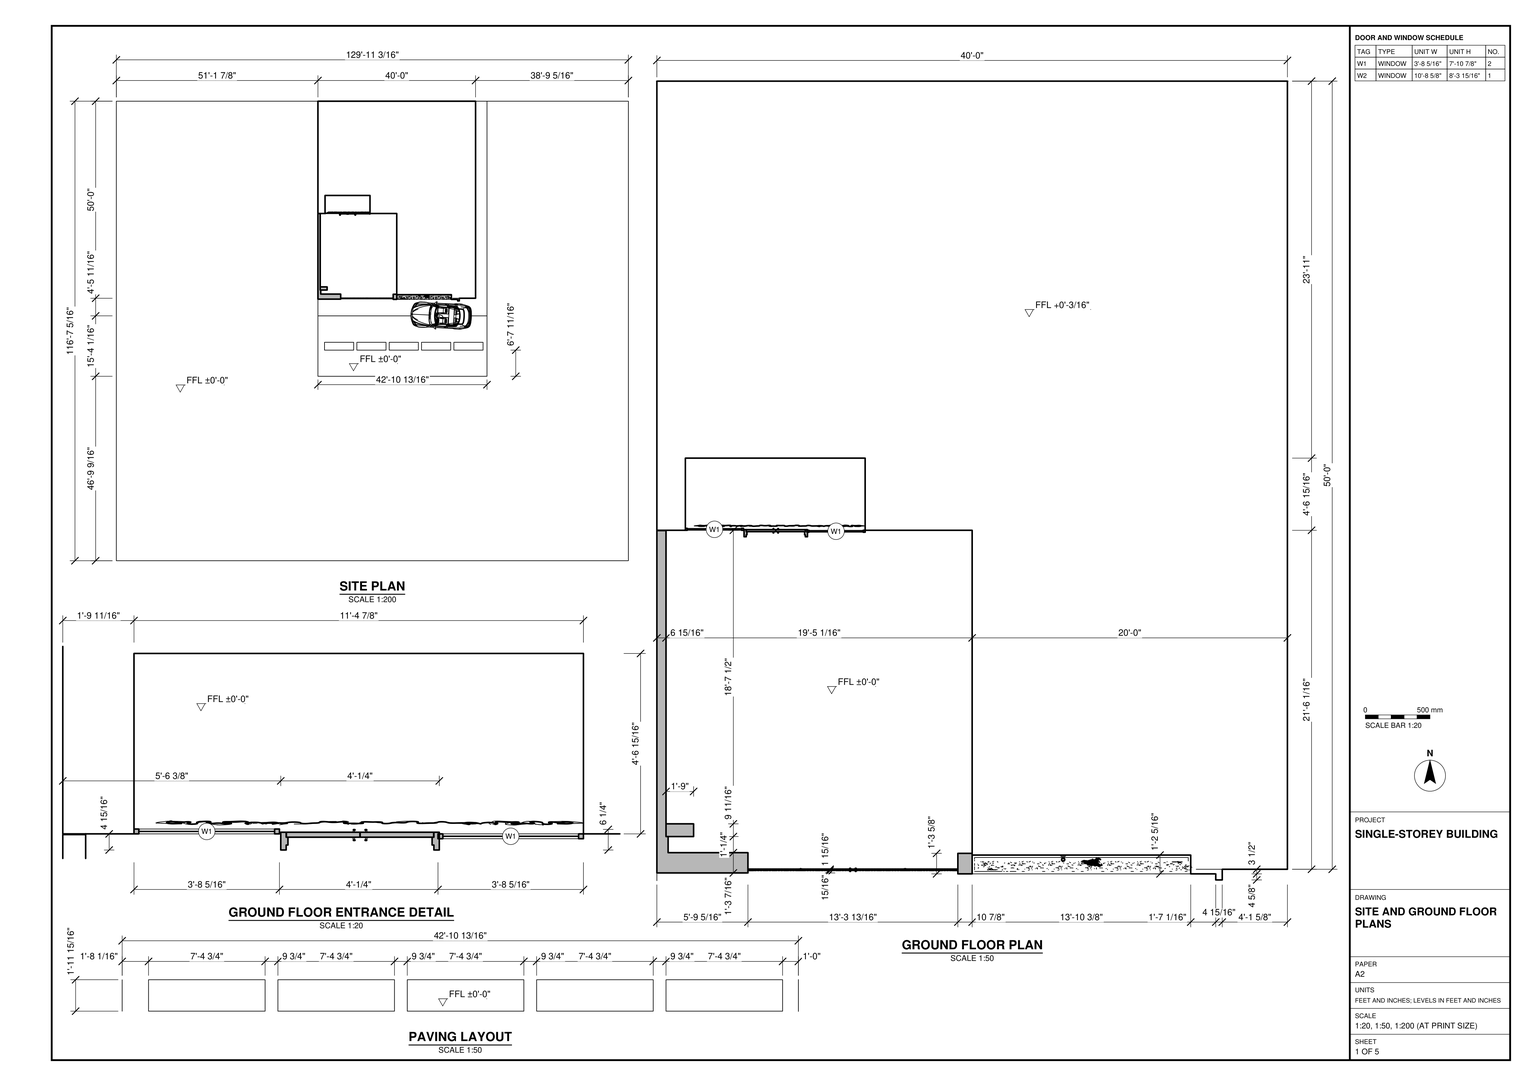
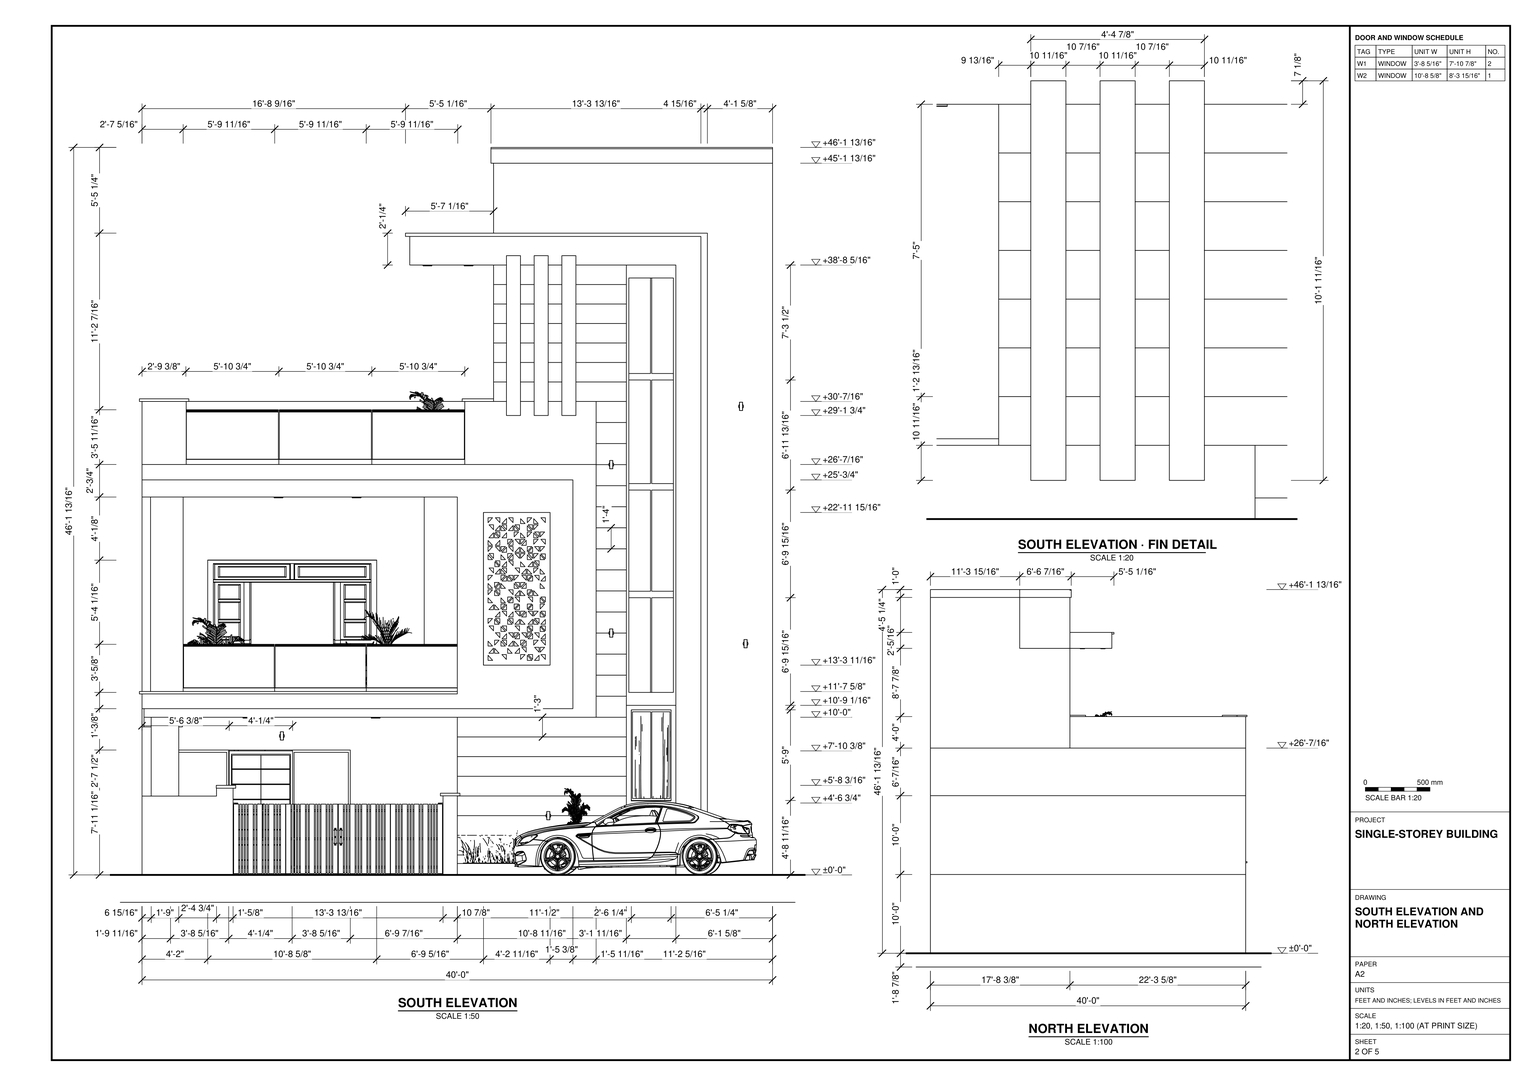
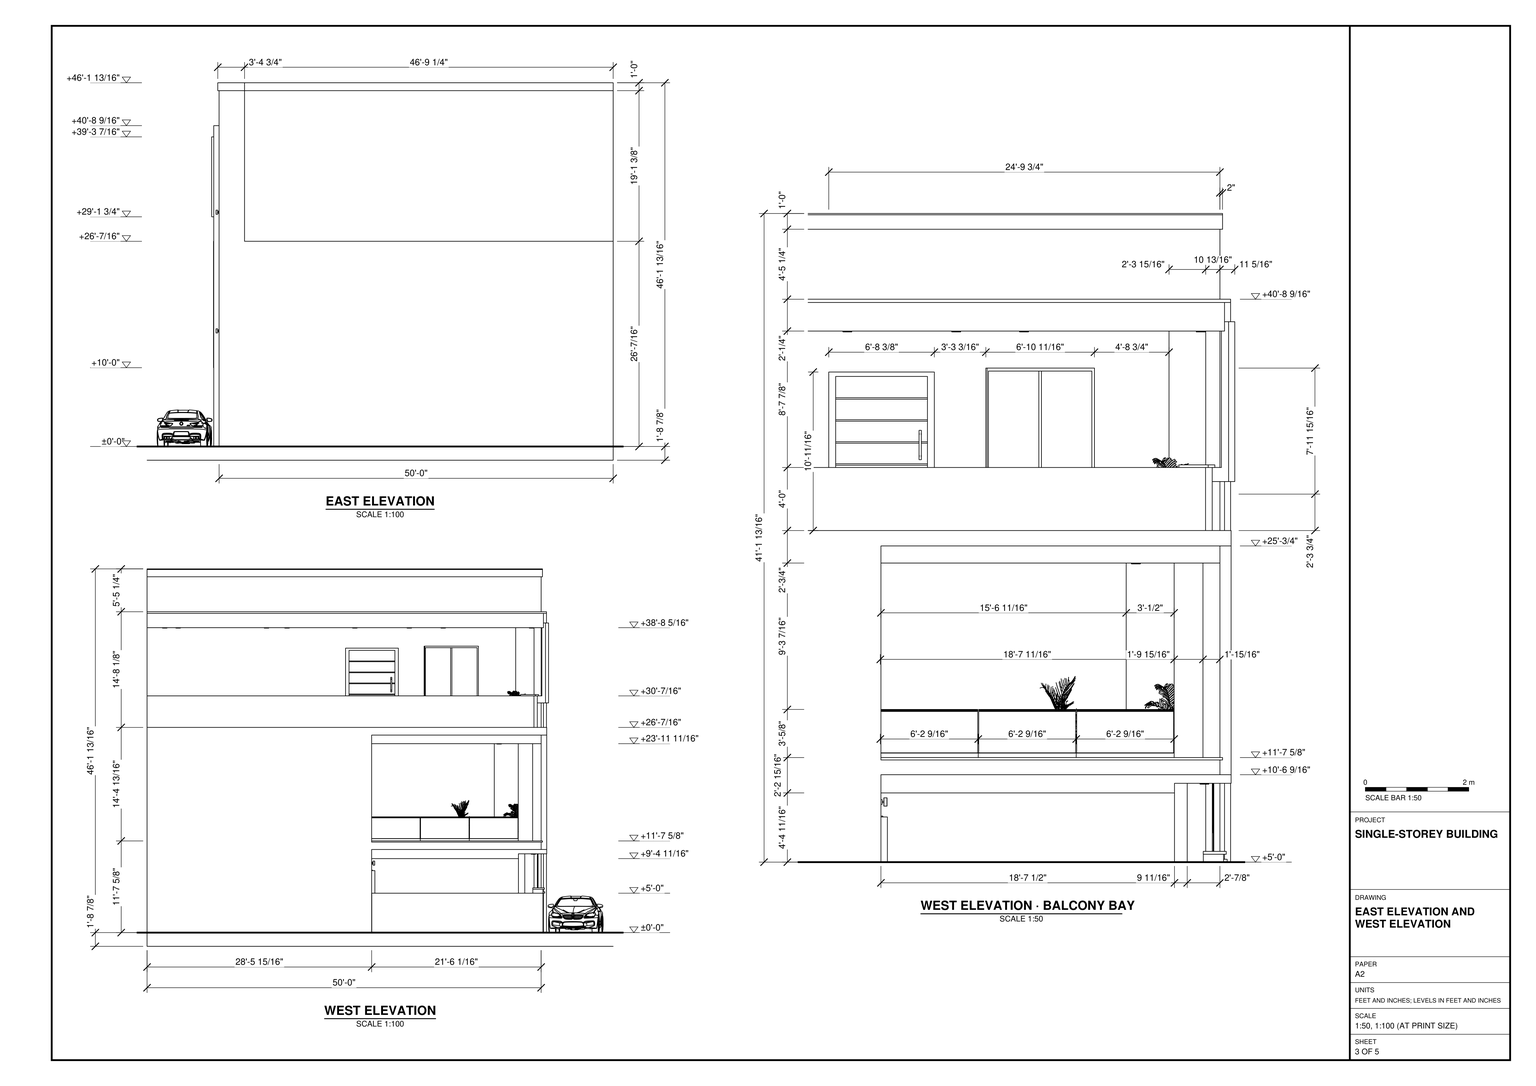
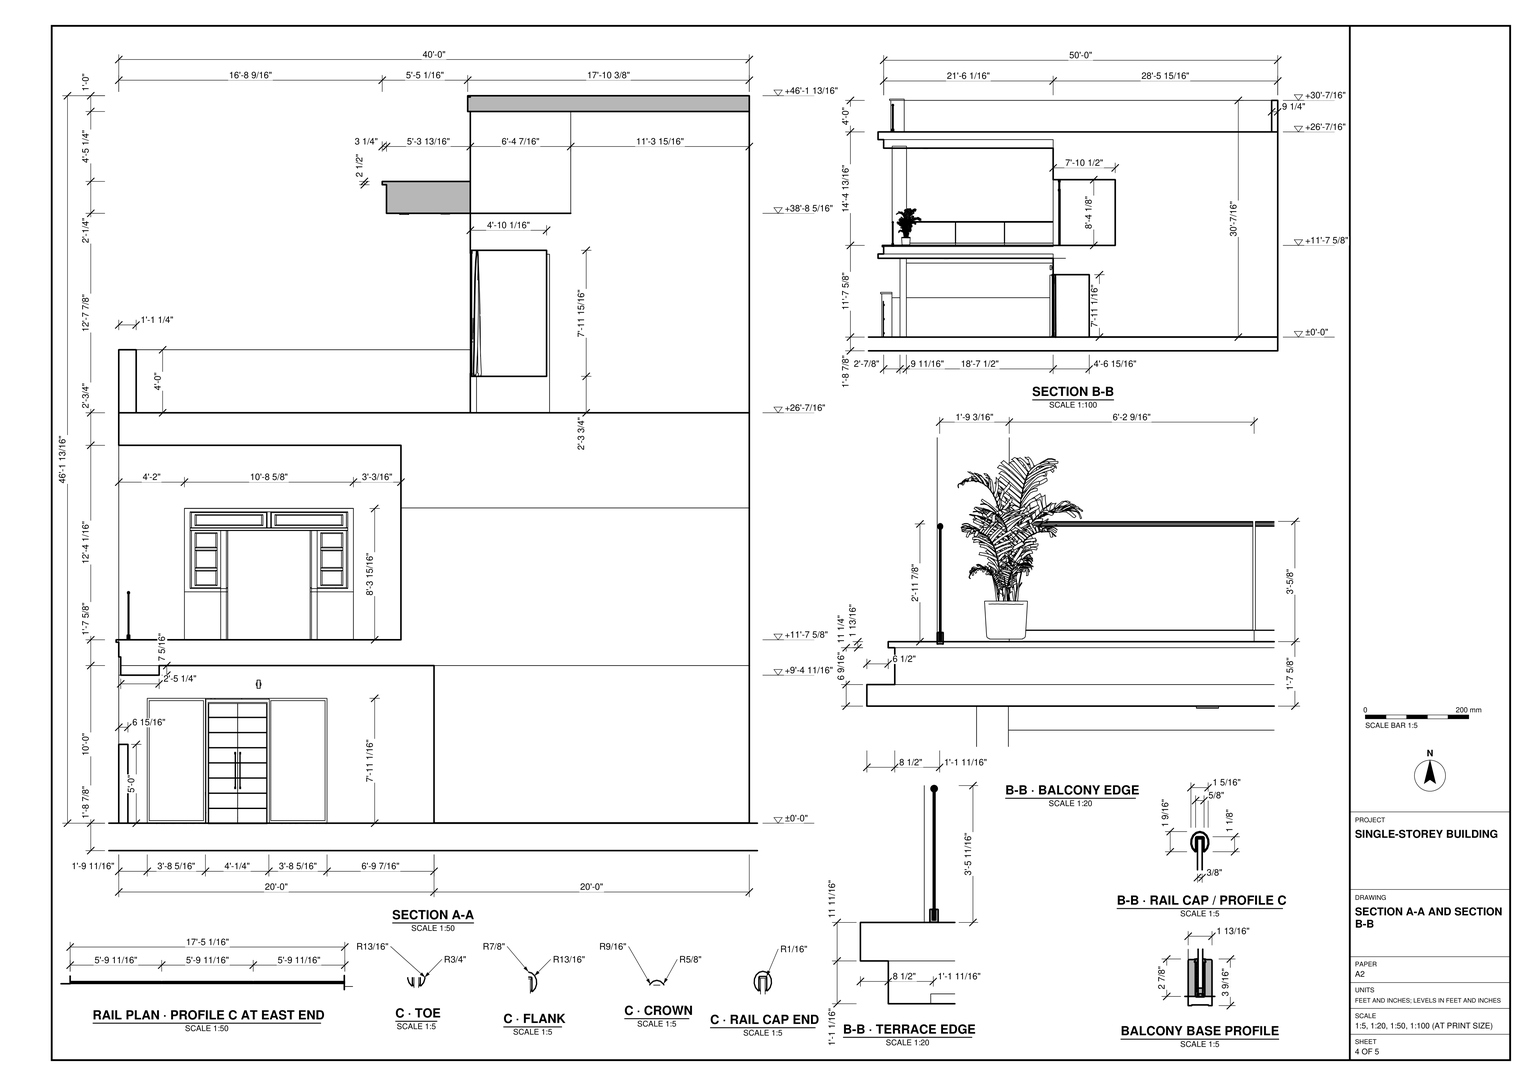
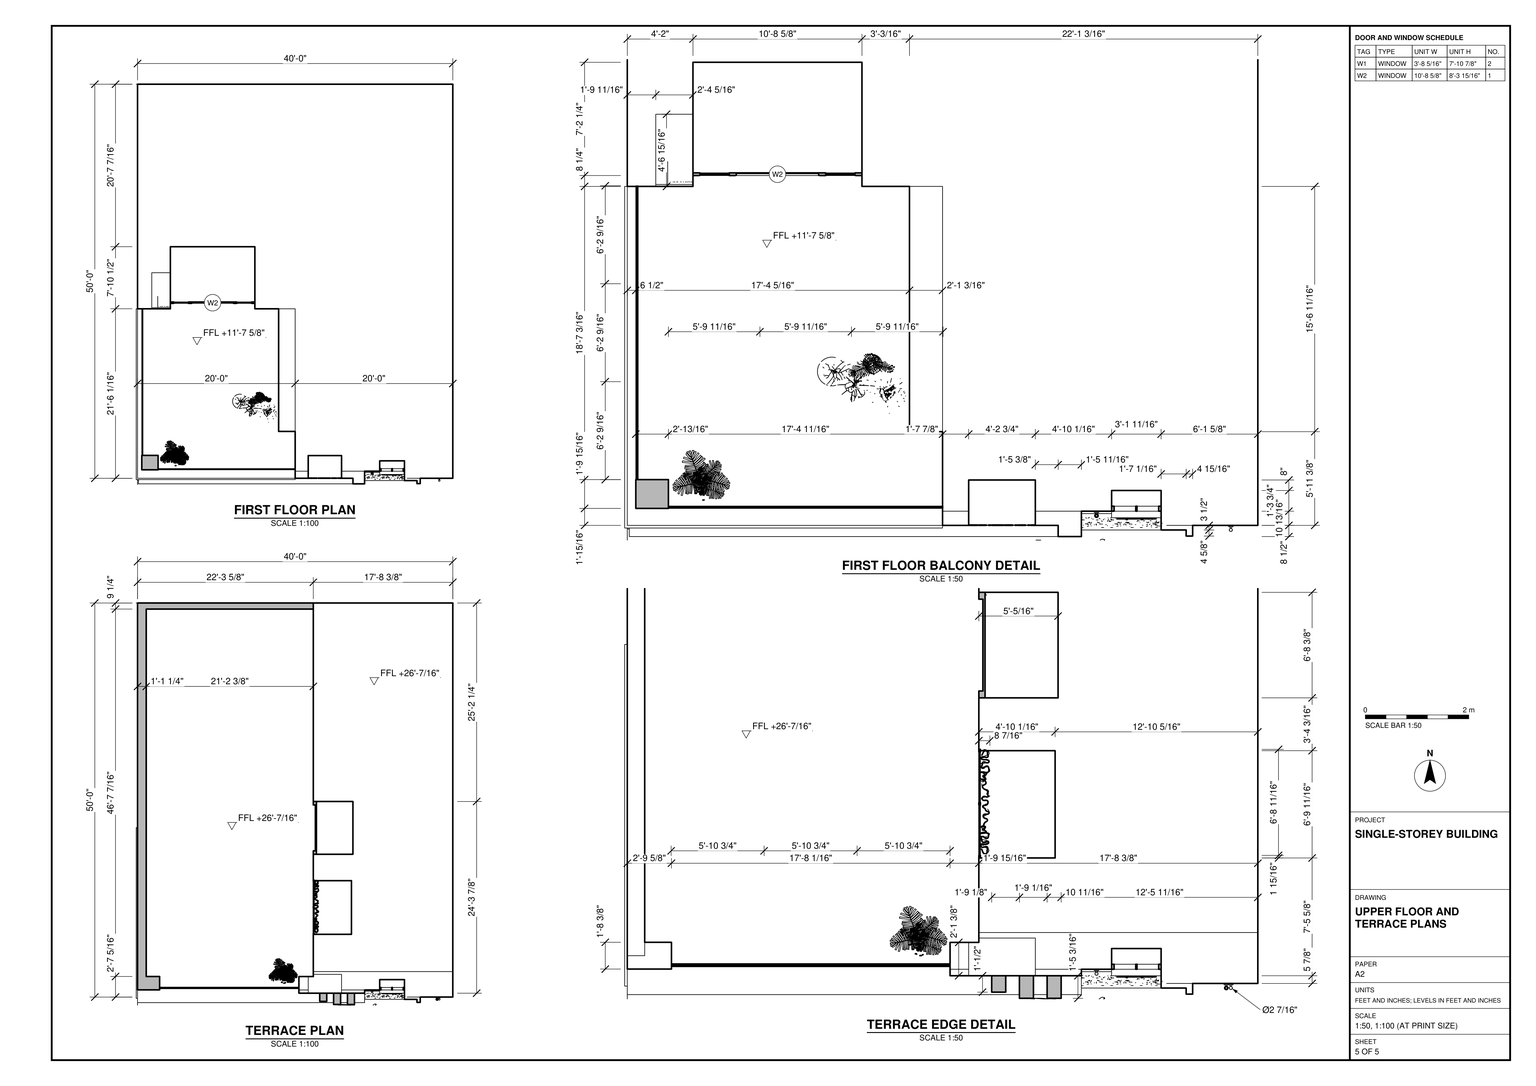
Build the house and its site in SketchUp from task_files/diagram_01.pdf. Work in feet and inches. The overall model measures 129'-11 3/16" along X, 116'-7 5/16" along Y and 47'-10 11/16" along Z. Use ±0'-0" as the ground-floor datum. Place the 40'-0" by 50'-0" building footprint against the north edge of the site, with the entrance facing south. Include the site base in the overall height; the highest roof cap is at +46'-1 13/16" relative to the ground floor.

Follow the plan for wall thicknesses, the recessed entrance, the window openings and the forecourt enclosure. Model the gate between its posts and the row of rectangular paving slabs in front. Use the south and west elevations together to set the depths of the balcony slabs, the returns of their railings and the roof projections. Reproduce the framed balcony opening, inset perforated screen, stepped flat roof, tall divided glazing and three projecting fins. Keep the east and north walls as plain as shown rather than carrying the south facade details around them.

Place the car and planting as shown; decor and loose items may be any suitable library components. Keep walls, slabs and roof elements in separate groups or components, do the same for each furniture or joinery piece, and use components for repeated parts. Save one SketchUp model as output_files/house_with_stacked_balconies_and_a_gated_forecourt.skp.

# SketchUp Ruby script. Lengths in inches.
U = 1.inch
M = Sketchup.active_model
def pt(a) = Geom::Point3d.new(a.map { |v| v * U })
def face(e, loops, mat)
  f = e.add_face(loops[0].map { |a| pt(a) })
  loops[1..].each { |l| e.add_face(l.map { |a| pt(a) }).erase! }
  f.material = f.back_material = mat if mat
  f
end
# faces: each face lists its corners as indices into pts; further lists are holes
def faces(e, pts, list, mat = nil) = list.each { |f| face(e, (f[0].is_a?(Array) ? f : [f]).map { |l| l.map { |i| pts[i] } }, mat) }
# xy, xz, yz: faces in a plane at the given z, y or x. An outline is a flat list of corners, or four numbers for a rectangle; further outlines are holes
def ring(l) = l.size == 4 ? [[l[0], l[1]], [l[2], l[1]], [l[2], l[3]], [l[0], l[3]]] : l.each_slice(2).to_a
def flat(e, list, mat, &to3) = list.each { |f| face(e, (f[0].is_a?(Array) ? f : [f]).map { |l| ring(l).map { |u, v| to3.(u, v) } }, mat) }
def xy(e, z, list, mat = nil) = flat(e, list, mat) { |x, y| [x, y, z] }
def xz(e, y, list, mat = nil) = flat(e, list, mat) { |x, z| [x, y, z] }
def yz(e, x, list, mat = nil) = flat(e, list, mat) { |y, z| [x, y, z] }
def lines(e, pts, list) = list.each { |a, b| e.add_line(pt(pts[a]), pt(pts[b])) }
# prism: a flat outline (further loops are holes) pulled along v
def prism(e, loops, v, mat = nil)
  f = face(e, loops, mat); d = Geom::Vector3d.new(v.map { |x| x * U })
  f.pushpull(f.normal.samedirection?(d) ? d.length : -d.length)
end
def box(e, o, s, mat = nil) = prism(e, [[o, [o[0] + s[0], o[1], o[2]], [o[0] + s[0], o[1] + s[1], o[2]], [o[0], o[1] + s[1], o[2]]]], [0, 0, s[2]], mat)
def at(x, y, z, deg = 0) = Geom::Transformation.translation(pt([x, y, z])) * Geom::Transformation.rotation(ORIGIN, Z_AXIS, deg.degrees)
def axes(o, x, y, z) = Geom::Transformation.new([*x, 0, *y, 0, *z, 0, *pt(o).to_a, 1])
def part(name) = M.definitions.add(name)
# library, detail: a bought-in or finely detailed component or shape, given as its bounding box
def library(name, o, s) = part(name).tap { |d| box(d.entities, o, s) }
def detail(e, o, s) = box(e.add_group.entities, o, s)
def put(e, d, t, mat = nil) = e.add_instance(d, t).tap { |i| i.material = mat if mat }
def group(e, t, mat = nil) = e.add_group.tap { |g| g.transformation = t; g.material = mat if mat }.entities
root = M.entities
M.materials.add("2").color = [128, 128, 128]
M.materials["2"].alpha = 0.5
M.materials.add("Material__1").color = [95, 70, 46]
M.materials.add("Material__2").color = [150, 168, 104]
M.materials.add("Material__3").color = [234, 233, 231]
M.materials.add("Material__4").color = [36, 36, 36]
M.materials.add("Material__5").color = [151, 172, 33]
M.materials.add("Material__6").color = [79, 108, 5]
M.materials.add("[0050_LemonChiffon]").color = [255, 250, 205]
M.materials.add("[0117_GhostWhite]").color = [248, 248, 255]
M.materials.add("[0131_Silver]").color = [192, 192, 192]
M.materials.add("[0132_LightGray]").color = [169, 169, 169]
M.materials.add("[0134_DimGray]").color = [105, 105, 105]
M.materials.add("[0135_DarkGray]").color = [81, 81, 81]
M.materials.add("[0137_Black]").color = [0, 0, 0]
M.materials.add("[Color M07]").color = [58, 58, 58]
M.materials.add("[Color_008]").color = [30, 30, 30]
M.materials.add("[Color_009]").color = [0, 0, 0]
M.materials.add("[Translucent Glass Gray]").color = [128, 128, 128]
M.materials["[Translucent Glass Gray]"].alpha = 0.5
M.materials.add("[Translucent Glass Gray]3").color = [128, 128, 128]
M.materials["[Translucent Glass Gray]3"].alpha = 0.3
M.materials.add("[Translucent_Glass_Gray]").color = [128, 128, 128]
M.materials["[Translucent_Glass_Gray]"].alpha = 0.5
M.materials.add("[Wood Bamboo]").color = [177, 105, 43]
M.materials.add("wire_1").color = [140, 184, 58]
M.materials.add("wire_2").color = [244, 244, 244]
M.materials.add("wire_4").color = [86, 225, 198]
M.materials.add("wire_5").color = [232, 232, 232]
c1 = library("Glass Railings(black Handrails)",[-57.04,-132.55,0],[169.29,2.52,28.17])
c2 = part("modern black window")
xy(c2.entities,0,[[0,-2,40,0]])
xy(c2.entities,2,[[2,-2,19.5,0],[19.5,-2,20.5,0],[20.5,-2,38,0]])
xy(c2.entities,16.625,[[2,-2,19.5,0],[20.5,-2,38,0]])
xy(c2.entities,17.625,[[2,-2,19.5,0],[20.5,-2,38,0]])
xy(c2.entities,33.25,[[2,-2,19.5,0],[20.5,-2,38,0]])
xy(c2.entities,34.25,[[2,-2,19.5,0],[20.5,-2,38,0]])
xy(c2.entities,50.25,[[2,-2,19.5,0],[20.5,-2,38,0]])
xy(c2.entities,51.25,[[2,-2,19.5,0],[20.5,-2,38,0]])
xy(c2.entities,66,[[2,-2,19.5,0],[19.5,-2,20,0],[20,-2,20.5,0],[20.5,-2,38,0]])
xy(c2.entities,68,[[0,-2,40,0]])
xz(c2.entities,-2,[[[0,0,40,68],[2,2,38,66]],[19.5,2,20.5,2,20.5,16.625,38,16.625,38,17.625,20.5,17.625,20.5,33.25,38,33.25,38,34.25,20.5,34.25,20.5,50.25,38,50.25,38,51.25,20.5,51.25,20.5,66,19.5,66,19.5,51.25,2,51.25,2,50.25,19.5,50.25,19.5,34.25,2,34.25,2,33.25,19.5,33.25,19.5,17.625,2,17.625,2,16.625,19.5,16.625]])
xz(c2.entities,0,[[[0,0,40,68],[2,2,38,66]],[19.5,2,19.5,16.625,2,16.625,2,17.625,19.5,17.625,19.5,33.25,2,33.25,2,34.25,19.5,34.25,19.5,50.25,2,50.25,2,51.25,19.5,51.25,19.5,66,20.5,66,20.5,51.25,38,51.25,38,50.25,20.5,50.25,20.5,34.25,38,34.25,38,33.25,20.5,33.25,20.5,17.625,38,17.625,38,16.625,20.5,16.625,20.5,2]])
yz(c2.entities,0,[[-2,0,0,68]])
yz(c2.entities,2,[[-2,2,0,16.625],[-2,16.625,0,17.625],[-2,17.625,0,33.25],[-2,33.25,0,34.25],[-2,34.25,0,34.5],
  [-2,34.5,0,50.25],[-2,50.25,0,51.25],[-2,51.25,0,66]])
yz(c2.entities,19.5,[[-2,2,0,16.625],[-2,17.625,0,33.25],[-2,34.25,0,50.25],[-2,51.25,0,66]])
yz(c2.entities,20.5,[[-2,2,0,16.625],[-2,17.625,0,33.25],[-2,34.25,0,50.25],[-2,51.25,0,66]])
yz(c2.entities,38,[[-2,2,0,16.625],[-2,16.625,0,17.625],[-2,17.625,0,33.25],[-2,33.25,0,34.25],[-2,34.25,0,50.25],
  [-2,50.25,0,51.25],[-2,51.25,0,66]])
yz(c2.entities,40,[[-2,0,0,68]])
c3 = library("Decorative grille panel",[0,0,0],[271.62,130.55,3])
c4 = library("window for srilanka",[-351.69,0,0],[94.49,3.9375,124.02])
c5 = part("WINDOW")
xy(c5.entities,0,[[0,0,59.06,1.97]],"[Color M07]")
xy(c5.entities,1.97,[[1.97,0,57.09,0.98],[1.97,0.98,57.09,1.97]],"[Color M07]")
xy(c5.entities,104.33,[[1.97,0,57.09,0.98],[1.97,0.98,57.09,1.97]],"[Color M07]")
xy(c5.entities,106.3,[[0,0,59.06,1.97]],"[Color M07]")
xz(c5.entities,0,[[[0,0,59.06,106.3],[1.97,1.97,57.09,104.33]]],"[Color M07]")
xz(c5.entities,0.98,[[1.97,1.97,57.09,104.33]],"[Translucent Glass Gray]3")
xz(c5.entities,1.97,[[[0,0,59.06,106.3],[1.97,1.97,57.09,104.33]]],"[Color M07]")
yz(c5.entities,0,[[0,0,1.97,106.3]],"[Color M07]")
yz(c5.entities,1.97,[[0,1.97,0.98,104.33],[0.98,1.97,1.97,104.33]],"[Color M07]")
yz(c5.entities,57.09,[[0,1.97,0.98,104.33],[0.98,1.97,1.97,104.33]],"[Color M07]")
yz(c5.entities,59.06,[[0,0,1.97,106.3]],"[Color M07]")
c6 = library("Component",[0,0,0],[11.41,86.61,113.31])
c7 = part("WindowDoubleBlack")
xy(c7.entities,0,[[0,0,96.0625,1.57]],"[0137_Black]")
xy(c7.entities,2.71,[[2.71,0,46.85,1.57],[49.41,0,93.35,1.57]],"[0137_Black]")
xy(c7.entities,122.09,[[2.71,0,46.85,1.57],[49.41,0,50,1.57],[50,0,93.35,1.57]],"[0137_Black]")
xy(c7.entities,124.8,[[0,0,96.0625,1.57]],"[0137_Black]")
xz(c7.entities,0,[[[0,0,96.0625,124.8],[2.71,2.71,46.85,122.09],[49.41,2.71,93.35,122.09]]],"[0137_Black]")
xz(c7.entities,1.57,[[2.71,2.71,46.85,122.09],[49.41,2.71,93.35,122.09]],"2")
xz(c7.entities,1.57,[[[0,0,96.0625,124.8],[2.71,2.71,46.85,122.09],[49.41,2.71,93.35,122.09]]],"[0137_Black]")
yz(c7.entities,0,[[0,0,1.57,124.8]],"[0137_Black]")
yz(c7.entities,2.71,[[0,2.71,1.57,122.09]],"[0137_Black]")
yz(c7.entities,46.85,[[0,2.71,1.57,122.09]],"[0137_Black]")
yz(c7.entities,49.41,[[0,2.71,1.57,122.09]],"[0137_Black]")
yz(c7.entities,93.35,[[0,2.71,1.57,122.09]],"[0137_Black]")
yz(c7.entities,96.0625,[[0,0,1.57,124.8]],"[0137_Black]")
c8 = library("Group5_1",[-7.56,-66.38,0.11],[6.33,135.04,120.95])
c9 = part("Group58\#1")
p = [[0,0,0],[0,0,-14.22],[-5.26,0,-14.22],[34.22,-11.8,0],[-34.22,-11.8,0],[34.22,11.8,0],
  [34.22,0,0],[-34.22,11.8,0],[5.26,0,-14.22],[-34.22,0,0],[0,0,-23.01]]
lines(c9.entities,p,[[0,1],[1,2],[3,4],[5,6],[7,5],[1,8],[9,0],[0,6],[8,10],[4,9],[6,3],[2,10],
  [9,7]])
c10 = part("Rectangle Light")
put(c10.entities,c9,at(0,0,0))
c11 = library("3 80",[0,-4.72,-0.01],[36.22,7.09,85.04])
c12 = part("Group65\#1")
p = [[0,0,0],[0,0,-10.18],[-3.34,0,-10.18],[21.74,-11.21,0],[-21.74,-11.21,0],[21.74,11.21,0],
  [21.74,0,0],[-21.74,11.21,0],[3.34,0,-10.18],[-21.74,0,0],[0,0,-16.47]]
lines(c12.entities,p,[[0,1],[1,2],[3,4],[5,6],[7,5],[1,8],[9,0],[0,6],[8,10],[4,9],[6,3],[2,10],
  [9,7]])
c13 = part("Rectangle Light\#1")
put(c13.entities,c12,at(0,0,0))
c14 = part("Janela")
xy(c14.entities,0,[[96.33,43.17,179.01,44.35]],"[Color_009]")
xy(c14.entities,1.97,[[98.3,44.15,136.6875,44.35],[138.66,44.15,177.04,44.35]])
xy(c14.entities,1.97,[[98.3,43.17,136.6875,43.46],[138.66,43.17,177.04,43.46]],"[Color_009]")
xy(c14.entities,80.71,[[98.3,43.17,136.6875,43.46],[138.66,43.17,177.04,43.46],[98.3,43.46,136.6875,44.15],[138.66,43.46,177.04,44.15],[98.3,44.15,136.6875,44.35],
  [138.66,44.15,177.04,44.35]])
xy(c14.entities,82.68,[[96.33,43.17,179.01,44.35]],"[Color_008]")
xz(c14.entities,43.17,[[[96.33,0,179.01,82.68],[98.3,1.97,136.6875,80.71],[138.66,1.97,177.04,80.71]]],"[Color_009]")
xz(c14.entities,43.46,[[98.3,1.97,136.6875,80.71],[138.66,1.97,177.04,80.71]],"[Translucent_Glass_Gray]")
xz(c14.entities,44.15,[[98.3,1.97,136.6875,80.71],[138.66,1.97,177.04,80.71]],"[Translucent_Glass_Gray]")
xz(c14.entities,44.35,[[[96.33,0,179.01,82.68],[98.3,1.97,177.04,80.71]],[136.6875,1.97,138.66,80.71]],"[Color_009]")
yz(c14.entities,96.33,[[43.17,0,44.35,82.68]],"[Color_009]")
yz(c14.entities,98.3,[[44.15,1.97,44.35,80.71]])
yz(c14.entities,98.3,[[43.17,1.97,43.46,80.71]],"[Color_009]")
yz(c14.entities,136.6875,[[43.17,1.97,43.46,80.71],[44.15,1.97,44.35,80.71]],"[Color_009]")
yz(c14.entities,138.66,[[43.17,1.97,43.46,80.71],[44.15,1.97,44.35,80.71]])
yz(c14.entities,177.04,[[43.17,1.97,43.46,80.71],[44.15,1.97,44.35,80.71]],"[Color_009]")
yz(c14.entities,179.01,[[43.17,0,44.35,82.68]],"[Color_009]")
c15 = library("Tlon Light 950 Ceiling 152 008",[-18.7,-18.7,-3.78],[37.4,37.4,3.56])
c16 = library("CONG SAT 05",[0,-2.03,0],[148.03,7.99,99.53])
c17 = library("House+plant_11",[37.27,36.97,0],[67.31,29.67,50.64])
c18 = library("KentiaPalm",[-22.86,-14.31,0],[47.49,43.96,59.125])
c19 = library("Group\#38",[-915.9375,-34.5,735.6],[41.04,40.85,6.81])
c20 = library("Group\#37",[-991.92,-34.05,729.49],[10.64,7.28,57.53])
c21 = library("Group\#36",[-1022.2,-71.69,736.68],[86.94,78.77,45.64])
c22 = library("Group\#35",[-877.77,-100.41,669.81],[37.9,37.9,42.75])
c23 = library("Group\#34",[-957.79,-83.08,701.98],[44.29,44.29,27.78])
c24 = library("Group\#33",[-1023.9,-65.47,669.625],[67.53,67.55,39.17])
c25 = library("Group\#32",[-997.48,-49.45,708.79],[29.81,29.81,30.61])
c26 = library("Group\#31",[-956738.95,-82059.81,669752.625],[42194.58,42232.57,49521.48])
c27 = library("Group\#30",[-917.52,-36.6875,711.84],[44.99,44.98,28.22])
c28 = library("Group\#29",[-916244.63,-35413.97,669800.48],[42442.38,42642.99,59706.29])
c29 = library("Group\#28",[-955.48,-54.29,730.4],[118.63,83.7,130.4])
c30 = library("Group\#27",[-899.97,-18.72,732.17],[8.78,8.27,28.64])
c31 = library("Group\#25",[-906.16,-138.28,686.8],[98.25,106.18,75.79])
c32 = library("Group\#24",[-978.71,-103.24,719.12],[90.2,76.4,68.29])
c33 = library("Group\#23",[-955.98,-81.17,725.57],[41.03,40.85,6.81])
c34 = library("Group\#21",[-996.8,-48.73,736.67],[28.51,28.38,4.73])
c35 = library("Group\#20",[-876.58,-99.29,706.19],[35.74,35.58,5.93])
c36 = library("Group\#18",[-912.1,-32.49,735.82],[33.14,36.63,9.55])
c37 = library("Group\#17",[-994.36,-46.95,735.88],[24.38,25.9,6.88])
c38 = part("PLANT-30")
p = [[0,0,0],[1,0,0],[1,1,0]]
lines(c38.entities,p,[[0,1],[1,2],[2,0]])
put(c38.entities,c19,at(895.63,-7.06,-669.82),"Material__1")
put(c38.entities,c20,at(895.63,-7.06,-669.82),"wire_1")
put(c38.entities,c21,at(895.63,-7.06,-669.82),"Material__2")
put(c38.entities,c22,at(895.63,-7.06,-669.82),"wire_2")
put(c38.entities,c23,at(895.63,-7.06,-669.82),"wire_2")
put(c38.entities,c24,at(895.63,-7.06,-669.82),"Material__3")
put(c38.entities,c25,at(895.63,-7.06,-669.82),"wire_2")
put(c38.entities,c26,axes([895.63,-7.06,-669.82],[0.001,0,0],[0,0.001,0],[0,0,0.001]),"Material__4")
put(c38.entities,c27,at(895.63,-7.06,-669.82),"wire_2")
put(c38.entities,c28,axes([895.63,-7.06,-669.82],[0.001,0,0],[0,0.001,0],[0,0,0.001]),"Material__4")
put(c38.entities,c29,at(895.63,-7.06,-669.82),"Material__5")
put(c38.entities,c30,at(895.63,-7.06,-669.82),"wire_4")
put(c38.entities,c31,at(895.63,-7.06,-669.82),"Material__6")
put(c38.entities,c32,at(895.63,-7.06,-669.82),"Material__4")
put(c38.entities,c33,at(895.63,-7.06,-669.82),"Material__1")
put(c38.entities,c34,at(895.63,-7.06,-669.82),"Material__1")
put(c38.entities,c35,at(895.63,-7.06,-669.82),"Material__1")
put(c38.entities,c36,at(895.63,-7.06,-669.82),"wire_5")
put(c38.entities,c37,at(895.63,-7.06,-669.82),"wire_5")
c39 = library("Lamp Wall Outdoor 94-02",[-1.89,-4.65,-3.17],[3.78,4.65,6.35])
c40 = library("car",[-8.95,-10.83,0],[83.51,184.88,55.74])
c41 = library("Dome Light",[-12,-12,0],[24,24,12])
xy(root,-21.0625,[[0,0,1559.1875,1399.3125]])
xy(root,-0.1875,[[0,0,1559.1875,0,1559.1875,1399.3125,1128.66,1399.3125,1128.66,561.5625,613.875,561.5625,613.875,1399.3125,0,1399.3125],[613.875,796.52,683.2,796.52,683.2,811.96,622.4375,811.96,622.4375,824.22,620.84,824.22,620.84,1057.15,613.875,1057.15]])
xy(root,-0.1875,[[633.95,641.24,722.7,665.17],[732.43,641.24,821.18,665.17],[830.92,641.24,919.67,665.17],[929.4,641.24,1018.15,665.17],[1027.89,641.24,1116.64,665.17],
  [613.875,745.6,1128.66,745.6,1128.66,1399.3125,613.875,1399.3125,613.875,1057.15,620.84,1057.15,620.84,833.9,641.84,833.9,641.84,824.22,622.4375,824.22,622.4375,811.96,683.2,811.96,683.2,796.52,613.875,796.52]],"[0050_LemonChiffon]")
xy(root,-0.1875,[[[613.875,561.5625,1128.66,745.6],[732.43,641.24,821.18,665.17],[830.92,641.24,919.67,665.17],[929.4,641.24,1018.15,665.17],[1027.89,641.24,1116.64,665.17],[633.95,641.24,722.7,665.17]]],"[Color_009]")
xy(root,0,[[1039.32,791.1875,1039.32,795.8125,1020.26,795.8125,1020.26,799.3125,1044.26,799.3125,1044.26,791.1875],[843,795.8125,853.875,811.4375],[[853.875,795.8125,1020.26,810.125],[855.72,797.66,1018.41,808.28]],[855.72,797.66,1018.41,808.28],[1020.26,799.3125,1093.875,799.3125,1093.875,1399.3125,613.875,1399.3125,613.875,1057.375,635.56,1057.375,635.56,1112.3125,772.41,1112.3125,772.41,1057.375,853.875,1057.375,853.875,810.125,1020.26,810.125]])
xy(root,8.5,[[[853.875,795.8125,1020.26,810.125],[855.72,797.66,1018.41,808.28]]],"[0117_GhostWhite]")
xy(root,52.45,[[982.57,805.125,1020.26,810.125]])
xy(root,56.16,[[986.29,805.125,1016.54,810.125]])
xy(root,59.8125,[[613.875,796.52,670.57,796.52,670.57,811.96,622.4375,811.96,622.4375,824.22,620.84,824.22,620.84,1057.15,613.875,1057.15]])
xy(root,60,[[841,793.8125,841,811.4375,843,811.4375,843,795.8125,853.875,795.8125,853.875,810.125,855.875,810.125,855.875,793.8125],[843,795.8125,853.875,811.4375]])
xy(root,62,[[841,793.8125,855.875,793.8125,855.875,810.125,853.875,810.125,853.875,811.4375,841,811.4375]],"[0135_DarkGray]")
xy(root,65.8125,[[670.38,794.52,685.2,796.52],[670.38,796.52,670.57,812.02],[670.57,796.52,683.2,811.96],[683.2,796.52,685.2,812.02],[670.57,811.96,683.2,812.02]])
xy(root,68,[[670.38,794.52,685.2,812.02]],"[0135_DarkGray]")
xy(root,94.88,[[635.56,1057.375,684.11,1112.3125],[684.11,1057.375,731.0625,1112.3125],[731.0625,1057.375,772.41,1112.3125]])
xy(root,112.5,[[615.375,833.9,644.63,1057.375]],"[0134_DimGray]")
xy(root,119.8125,[[615.375,790.8125,615.375,833.9,620.84,833.9,620.84,824.22,641.84,824.22,641.84,833.9,644.63,833.9,644.63,1057.375,853.875,1057.375,853.875,810.125,959.5625,810.125,959.5625,790.8125]])
xy(root,125.17,[[986.29,805.125,1016.54,810.125]])
xy(root,126.375,[[615.375,790.8125,941.88,799.3125],[613.875,799.3125,615.375,833.9],[613.875,833.9,615.375,1057.375]])
xy(root,128.88,[[982.57,805.125,1020.26,825.875]])
xy(root,137.59,[[611.875,797.3125,611.875,1057.375,613.875,1057.375,613.875,799.3125,853.875,799.3125,853.875,797.3125]])
xy(root,139.4375,[[611.875,797.3125,853.875,797.3125,853.875,799.3125,613.875,799.3125,613.875,1057.375,611.875,1057.375],[[613.875,799.3125,853.875,799.3125,853.875,870.66,828.6875,870.66,828.6875,1057.375,792.52,1057.375,792.52,1065.64,663.87,1065.64,663.87,1057.375,613.875,1057.375],[620.36,812.23,645.17,834.17]]])
xy(root,139.4375,[[691.48,1065.64,764.91,1065.64,764.91,1067.6875,792.52,1067.6875,792.52,1151.875,663.87,1151.875,663.87,1067.6875,691.48,1067.6875]],"[0134_DimGray]")
xy(root,159.49,[[873.75,799.3125,924.5,833.875]])
xy(root,175.93,[[663.87,1065.64,691.48,1067.6875],[764.91,1065.64,792.52,1067.6875]])
xy(root,239.53,[[663.87,1057.375,792.52,1151.875]])
xy(root,275.74,[[873.75,799.3125,924.5,833.875]])
xy(root,287.5,[[613.875,799.3125,613.875,1057.375,828.6875,1057.375,828.6875,870.66,853.875,870.66,853.875,799.3125]])
xy(root,290.5,[[620.36,812.23,645.17,834.17]])
xy(root,300.53,[[613.875,790.8125,941.88,799.3125]])
xy(root,312.25,[[613.875,790.8125,959.5625,790.8125,959.5625,805.1875,859.58,805.1875,859.58,830.5625,881.5,830.5625,881.5,1016.72,941.8125,1016.72,941.8125,1097.08,881.5,1097.08,881.5,1390.05,627.13,1390.05,627.13,830.63,647.51,830.63,647.51,810.26,613.875,810.26],[613.875,810.26,647.51,810.26,647.51,830.63,627.13,830.63,627.13,820.45,613.875,820.45],[613.875,820.45,613.875,1399.3125,881.5,1399.3125,881.5,1390.05,627.13,1390.05,627.13,820.45],[881.5,838.0625,1093.875,838.0625,1093.875,1399.3125,881.5,1399.3125,881.5,1097.08,941.8125,1097.08,941.8125,1016.72,881.5,1016.72]])
xy(root,340,[[881.5,894.84,939.5625,976.53]])
xy(root,349.5625,[[912.375,788,923.0625,805.1875],[933.47,788,944.16,805.1875],[891.28,792.6875,901.97,805.1875]],"[0134_DimGray]")
xy(root,360.25,[[891.28,798.1875,901.97,805.1875],[912.375,798.1875,923.0625,805.1875],[933.47,798.1875,944.16,805.1875],[859.58,805.1875,881.5,830.5625],[881.5,805.1875,959.5625,810.125],
  [611.875,810.26,613.875,830.63],[613.875,810.26,647.51,830.63],[613.875,830.63,627.13,830.63,627.13,1390.05,881.5,1390.05,881.5,1399.3125,613.875,1399.3125]])
xy(root,360.25,[[857.58,803.1875,881.5,805.1875],[857.58,805.1875,859.58,830.5625],[611.875,808.26,647.51,810.26],[647.51,808.26,649.51,830.63]],"[0132_LightGray]")
xy(root,362.25,[[857.58,803.1875,881.5,830.5625],[611.875,808.26,649.51,830.63]],"[0132_LightGray]")
xy(root,432.9375,[[881.5,1016.72,941.8125,1097.08]])
xy(root,435.9375,[[881.5,894.84,939.5625,976.53]])
xy(root,464.1,[[817.6875,795.8125,817.6875,1399.3125,957.9375,1399.3125,957.9375,810.125,982.57,810.125,982.57,825.875,1020.26,825.875,1020.26,795.8125]])
xy(root,471.25,[[912.375,788,923.0625,798.1875],[933.47,788,944.16,798.1875],[891.28,792.6875,901.97,798.1875]],"[0134_DimGray]")
xy(root,485.875,[[814.4375,791.1875,814.4375,1399.3125,817.6875,1399.3125,817.6875,795.8125,1039.32,795.8125,1039.32,791.1875]],"[0134_DimGray]")
xy(root,488.375,[[814.4375,791.1875,1044.26,791.1875,1044.26,799.3125,881.5,799.3125,881.5,1399.3125,814.4375,1399.3125]])
xy(root,541.625,[[879.5,797.3125,1093.875,799.3125],[879.5,799.3125,881.5,1399.3125],[881.5,799.3125,1093.875,1399.3125]])
xy(root,552.625,[[879.5,797.3125,881.5,799.3125],[879.5,799.3125,881.5,1399.3125]])
xy(root,553.625,[[879.5,797.3125,1093.875,1399.3125]])
xz(root,0,[[0,-21.0625,1559.1875,-0.1875]])
xz(root,788,[[912.375,349.5625,923.0625,471.25],[933.47,349.5625,944.16,471.25]],"[0134_DimGray]")
xz(root,790.8125,[[615.375,119.8125,959.5625,119.8125,959.5625,312.25,613.875,312.25,613.875,300.53,941.88,300.53,941.88,126.375,615.375,126.375]])
xz(root,791.1875,[[1039.32,0,1044.26,0,1044.26,488.375,814.4375,488.375,814.4375,485.875,1039.32,485.875]],"[0134_DimGray]")
xz(root,792.6875,[[891.28,349.5625,901.97,471.25]],"[0134_DimGray]")
xz(root,793.8125,[[841,60,855.875,62]],"[0135_DarkGray]")
xz(root,794.52,[[670.38,65.8125,685.2,68]],"[0135_DarkGray]")
xz(root,795.8125,[[1020.26,0,1039.32,0,1039.32,485.875,817.6875,485.875,817.6875,464.1,1020.26,464.1],[843,0,853.875,60]])
xz(root,795.8125,[[853.875,0,1020.26,8.5]],"[0117_GhostWhite]")
xz(root,796.52,[[613.875,-0.1875,683.2,-0.1875,683.2,65.8125,670.57,65.8125,670.57,59.8125,613.875,59.8125]])
xz(root,797.3125,[[611.875,137.59,853.875,139.4375],[879.5,541.625,1093.875,552.625]])
xz(root,797.3125,[[879.5,552.625,1093.875,553.625]],"[0134_DimGray]")
xz(root,797.66,[[855.72,0,1018.41,8.5]])
xz(root,798.1875,[[891.28,360.25,901.97,471.25],[912.375,360.25,923.0625,471.25],[933.47,360.25,944.16,471.25]])
xz(root,799.3125,[[1044.26,-0.1875,1093.875,0],[[613.875,126.375,941.88,126.375,941.88,300.53,613.875,300.53,613.875,287.5,853.875,287.5,853.875,137.59,613.875,137.59],[873.75,159.49,924.5,275.74]]])
xz(root,799.3125,[[1044.26,0,1093.875,0,1093.875,541.625,881.5,541.625,881.5,488.375,1044.26,488.375]],"[0131_Silver]")
xz(root,803.1875,[[857.58,360.25,881.5,362.25]],"[0132_LightGray]")
xz(root,805.125,[[[982.57,52.45,1020.26,128.88],[986.29,56.16,1016.54,125.17]]])
xz(root,805.1875,[[859.58,312.25,959.5625,312.25,959.5625,360.25,944.16,360.25,944.16,349.5625,933.47,349.5625,933.47,360.25,923.0625,360.25,923.0625,349.5625,912.375,349.5625,912.375,360.25,901.97,360.25,901.97,349.5625,891.28,349.5625,891.28,360.25,859.58,360.25],[891.28,349.5625,901.97,360.25],[912.375,349.5625,923.0625,360.25],[933.47,349.5625,944.16,360.25]])
xz(root,808.26,[[611.875,360.25,649.51,362.25]],"[0132_LightGray]")
xz(root,808.28,[[855.72,0,1018.41,8.5]],"[0117_GhostWhite]")
xz(root,810.125,[[853.875,0,1020.26,8.5],[986.29,56.16,1016.54,59.91],[986.29,59.91,1016.54,74.88],[853.875,60,855.875,62],[986.29,74.88,1016.54,89.86],
  [986.29,89.86,1016.54,104.84],[986.29,104.84,1016.54,119.8125],[986.29,119.8125,1016.54,125.17],[881.5,464.1,957.9375,488.375]])
xz(root,810.125,[[853.875,8.5,1020.26,14.98],[853.875,14.98,1020.26,29.95],[853.875,29.95,1020.26,44.93],[853.875,44.93,1020.26,44.93,1020.26,52.45,982.57,52.45,982.57,59.91,853.875,59.91],[853.875,59.91,982.57,59.91,982.57,74.88,853.875,74.88,853.875,62,855.875,62,855.875,60,853.875,60],
  [853.875,74.88,982.57,89.86],[853.875,89.86,982.57,104.84],[853.875,104.84,982.57,119.8125],[959.5625,119.8125,982.57,135.84],[959.5625,135.84,982.57,151.87],
  [959.5625,151.87,982.57,167.9],[959.5625,167.9,982.57,183.93],[959.5625,183.93,982.57,199.96],[959.5625,199.96,982.57,215.99],[959.5625,215.99,982.57,232.02],
  [959.5625,232.02,982.57,248.05],[959.5625,248.05,982.57,264.08],[959.5625,264.08,982.57,280.1],[959.5625,280.1,982.57,296.13],[959.5625,296.13,982.57,312.16],
  [959.5625,312.16,982.57,328.19],[959.5625,328.19,982.57,344.22],[959.5625,344.22,982.57,360.25],[881.5,360.25,982.57,375.09],[881.5,375.09,982.57,389.92],
  [881.5,389.92,982.57,404.76],[881.5,404.76,982.57,419.6],[881.5,419.6,982.57,434.43],[881.5,434.43,982.57,449.27],[881.5,449.27,982.57,464.1]],"[Wood Bamboo]")
xz(root,810.26,[[613.875,312.25,647.51,360.25]])
xz(root,811.4375,[[843,0,853.875,60]])
xz(root,811.4375,[[841,60,843,62],[843,60,853.875,62]],"[0135_DarkGray]")
xz(root,811.96,[[622.4375,-0.1875,622.4375,59.8125,670.57,59.8125,670.57,65.8125,683.2,65.8125,683.2,-0.1875]])
xz(root,812.02,[[670.38,65.8125,685.2,68]],"[0135_DarkGray]")
xz(root,812.23,[[620.36,139.4375,645.17,290.5]],"[0134_DimGray]")
xz(root,824.22,[[620.84,-0.1875,622.4375,59.8125],[622.4375,-0.1875,641.84,-0.1875,641.84,119.8125,620.84,119.8125,620.84,59.8125,622.4375,59.8125]],"[0134_DimGray]")
xz(root,825.875,[[982.57,128.88,1020.26,464.1]])
xz(root,830.5625,[[859.58,312.25,881.5,360.25],[857.58,360.25,881.5,362.25]])
xz(root,830.63,[[627.13,312.25,647.51,360.25],[611.875,360.25,627.13,362.25],[627.13,360.25,649.51,362.25]])
xz(root,833.875,[[873.75,159.49,924.5,275.74]])
xz(root,833.9,[[620.84,-0.1875,641.84,112.5],[615.375,112.5,620.84,119.8125],[641.84,112.5,644.63,119.8125]],"[0134_DimGray]")
xz(root,834.17,[[620.36,139.4375,645.17,290.5]],"[0134_DimGray]")
xz(root,870.66,[[828.6875,139.4375,853.875,287.5]],"[0050_LemonChiffon]")
xz(root,894.84,[[881.5,340,939.5625,435.9375]])
xz(root,976.53,[[881.5,340,939.5625,435.9375]])
xz(root,1016.72,[[881.5,312.25,941.8125,432.9375]])
xz(root,1057.15,[[613.875,-0.1875,620.84,59.8125]])
xz(root,1057.375,[[613.875,112.5,615.375,126.375],[611.875,137.59,613.875,139.4375]])
xz(root,1057.375,[[613.875,0,635.56,0,635.56,94.88,772.41,94.88,772.41,0,853.875,0,853.875,119.8125,644.63,119.8125,644.63,112.5,613.875,112.5],[613.875,139.4375,663.87,139.4375,663.87,239.53,792.52,239.53,792.52,139.4375,828.6875,139.4375,828.6875,287.5,613.875,287.5]],"[0050_LemonChiffon]")
xz(root,1065.64,[[663.87,139.4375,691.48,175.93],[764.91,139.4375,792.52,175.93]],"[Translucent Glass Gray]")
xz(root,1067.6875,[[663.87,139.4375,691.48,175.93],[764.91,139.4375,792.52,175.93]])
xz(root,1097.08,[[881.5,312.25,941.8125,432.9375]])
xz(root,1112.3125,[[635.56,0,684.11,94.88],[684.11,0,731.0625,94.88],[731.0625,0,772.41,94.88]])
xz(root,1151.875,[[663.87,139.4375,792.52,239.53]])
xz(root,1390.05,[[627.13,312.25,881.5,360.25]])
xz(root,1399.3125,[[0,-21.0625,1559.1875,-0.1875],[613.875,-0.1875,1093.875,0],[613.875,0,1093.875,119.8125],[613.875,119.8125,1093.875,239.8125],[613.875,239.8125,1093.875,312.25],
  [613.875,312.25,881.5,360.25],[881.5,312.25,881.5,464.1,957.9375,464.1,957.9375,541.625,1093.875,541.625,1093.875,312.25],[817.6875,464.1,881.5,488.375],[881.5,464.1,957.9375,541.625],[814.4375,485.875,817.6875,488.375],
  [879.5,541.625,879.5,552.625,881.5,552.625,881.5,553.625,957.9375,553.625,957.9375,541.625],[957.9375,541.625,1093.875,553.625],[879.5,552.625,881.5,553.625]])
yz(root,0,[[0,-21.0625,1399.3125,-0.1875]])
yz(root,611.875,[[797.3125,137.59,1057.375,139.4375]])
yz(root,611.875,[[808.26,360.25,830.63,362.25]],"[0132_LightGray]")
yz(root,613.875,[[796.52,-0.1875,1057.15,59.8125],[1057.375,0,1057.375,126.375,799.3125,126.375,799.3125,137.59,1057.375,137.59,1057.375,300.53,790.8125,300.53,790.8125,312.25,1399.3125,312.25,1399.3125,0],[799.3125,287.5,1057.375,300.53],[810.26,312.25,1399.3125,360.25]])
yz(root,615.375,[[833.9,112.5,833.9,119.8125,790.8125,119.8125,790.8125,126.375,1057.375,126.375,1057.375,112.5]],"[0134_DimGray]")
yz(root,620.36,[[812.23,139.4375,834.17,290.5]],"[0134_DimGray]")
yz(root,620.84,[[833.9,-0.1875,1057.15,59.8125]])
yz(root,620.84,[[824.22,-0.1875,833.9,59.8125],[824.22,59.8125,833.9,119.8125]],"[0134_DimGray]")
yz(root,622.4375,[[811.96,-0.1875,824.22,59.8125]])
yz(root,627.13,[[830.63,312.25,1390.05,360.25]])
yz(root,635.56,[[1057.375,0,1112.3125,94.88]])
yz(root,641.84,[[824.22,-0.1875,833.9,119.8125]],"[0134_DimGray]")
yz(root,644.63,[[833.9,112.5,1057.375,119.8125]],"[0134_DimGray]")
yz(root,645.17,[[812.23,139.4375,834.17,290.5]],"[0134_DimGray]")
yz(root,647.51,[[810.26,312.25,830.63,360.25]])
yz(root,649.51,[[808.26,360.25,830.63,362.25]],"[0132_LightGray]")
yz(root,663.87,[[1057.375,139.4375,1065.64,139.4375,1065.64,175.93,1067.6875,175.93,1067.6875,139.4375,1151.875,139.4375,1151.875,239.53,1057.375,239.53]])
yz(root,670.38,[[794.52,65.8125,812.02,68]],"[0135_DarkGray]")
yz(root,670.57,[[796.52,59.8125,811.96,65.8125]])
yz(root,683.2,[[796.52,-0.1875,811.96,65.8125]])
yz(root,685.2,[[794.52,65.8125,812.02,68]],"[0135_DarkGray]")
yz(root,691.48,[[1065.64,139.4375,1067.6875,175.93]])
yz(root,764.91,[[1065.64,139.4375,1067.6875,175.93]])
yz(root,772.41,[[1057.375,0,1112.3125,94.88]])
yz(root,792.52,[[1057.375,139.4375,1057.375,239.53,1151.875,239.53,1151.875,139.4375,1067.6875,139.4375,1067.6875,175.93,1065.64,175.93,1065.64,139.4375]])
yz(root,814.4375,[[791.1875,485.875,1399.3125,488.375]],"[0134_DimGray]")
yz(root,817.6875,[[795.8125,464.1,1399.3125,485.875]])
yz(root,828.6875,[[870.66,139.4375,1057.375,287.5]],"[0050_LemonChiffon]")
yz(root,841,[[793.8125,60,811.4375,62]],"[0135_DarkGray]")
yz(root,843,[[795.8125,0,811.4375,60]])
yz(root,853.875,[[795.8125,0,810.125,8.5],[795.8125,8.5,810.125,60],[810.125,60,811.4375,62],[797.3125,137.59,799.3125,139.4375]])
yz(root,853.875,[[810.125,0,811.4375,60],[811.4375,0,811.4375,62,810.125,62,810.125,119.8125,1057.375,119.8125,1057.375,0],[799.3125,139.4375,870.66,287.5]],"[0050_LemonChiffon]")
yz(root,855.72,[[797.66,0,808.28,8.5]])
yz(root,855.875,[[793.8125,60,810.125,62]])
yz(root,857.58,[[803.1875,360.25,830.5625,362.25]],"[0132_LightGray]")
yz(root,859.58,[[805.1875,312.25,830.5625,360.25]])
yz(root,873.75,[[799.3125,159.49,833.875,275.74]])
yz(root,879.5,[[797.3125,541.625,1399.3125,552.625]])
yz(root,879.5,[[797.3125,552.625,1399.3125,553.625]],"[0134_DimGray]")
yz(root,881.5,[[1390.05,312.25,1399.3125,360.25],[803.1875,360.25,810.125,362.25],[810.125,360.25,830.5625,362.25]])
yz(root,881.5,[[830.5625,312.25,830.5625,362.25,810.125,362.25,810.125,488.375,838.0625,488.375,838.0625,312.25],[[838.0625,312.25,838.0625,488.375,1399.3125,488.375,1399.3125,360.25,1390.05,360.25,1390.05,312.25,1097.08,312.25,1097.08,432.9375,1016.72,432.9375,1016.72,312.25],[894.84,340,976.53,435.9375]]],"[0050_LemonChiffon]")
yz(root,881.5,[[799.3125,488.375,1399.3125,541.625]],"[0131_Silver]")
yz(root,891.28,[[792.6875,349.5625,792.6875,471.25,798.1875,471.25,798.1875,360.25,805.1875,360.25,805.1875,349.5625]],"[0134_DimGray]")
yz(root,901.97,[[792.6875,349.5625,805.1875,349.5625,805.1875,360.25,798.1875,360.25,798.1875,471.25,792.6875,471.25]],"[0134_DimGray]")
yz(root,912.375,[[788,349.5625,788,471.25,798.1875,471.25,798.1875,360.25,805.1875,360.25,805.1875,349.5625]],"[0134_DimGray]")
yz(root,923.0625,[[788,349.5625,805.1875,349.5625,805.1875,360.25,798.1875,360.25,798.1875,471.25,788,471.25]],"[0134_DimGray]")
yz(root,924.5,[[799.3125,159.49,833.875,275.74]])
yz(root,933.47,[[788,349.5625,788,471.25,798.1875,471.25,798.1875,360.25,805.1875,360.25,805.1875,349.5625]],"[0134_DimGray]")
yz(root,939.5625,[[894.84,340,976.53,435.9375]])
yz(root,941.8125,[[1016.72,312.25,1097.08,432.9375]])
yz(root,941.88,[[790.8125,126.375,799.3125,300.53]])
yz(root,944.16,[[788,349.5625,805.1875,349.5625,805.1875,360.25,798.1875,360.25,798.1875,471.25,788,471.25]],"[0134_DimGray]")
yz(root,959.5625,[[790.8125,119.8125,810.125,312.25],[805.1875,312.25,810.125,360.25]])
yz(root,982.57,[[805.125,52.45,810.125,128.88],[810.125,128.88,825.875,464.1]])
yz(root,986.29,[[805.125,56.16,810.125,125.17]])
yz(root,1016.54,[[805.125,56.16,810.125,125.17]])
yz(root,1018.41,[[797.66,0,799.3125,8.5],[799.3125,0,808.28,8.5]])
yz(root,1020.26,[[795.8125,0,799.3125,8.5],[799.3125,0,810.125,8.5],[795.8125,8.5,799.3125,464.1],[799.3125,8.5,799.3125,464.1,825.875,464.1,825.875,128.88,805.125,128.88,805.125,52.45,810.125,52.45,810.125,8.5]])
yz(root,1039.32,[[791.1875,0,795.8125,485.875]],"[0134_DimGray]")
yz(root,1044.26,[[791.1875,0,799.3125,488.375]],"[0134_DimGray]")
yz(root,1093.875,[[799.3125,-0.1875,1399.3125,0],[799.3125,0,1399.3125,0,1399.3125,312.25,838.0625,312.25,838.0625,541.625,799.3125,541.625],[838.0625,312.25,1399.3125,541.625],[797.3125,541.625,838.0625,553.625],[838.0625,541.625,1399.3125,553.625]])
yz(root,1559.1875,[[0,-21.0625,1399.3125,-0.1875]])
p = [[613.875,799.3125,-0.1875],[613.875,799.3125,0],[957.9375,799.3125,464.1],[957.9375,799.3125,488.375],[982.57,810.125,59.91],[986.29,810.125,59.91],
  [1016.54,810.125,59.91],[1020.26,810.125,59.91],[982.57,810.125,74.88],[986.29,810.125,74.88],[1016.54,810.125,74.88],[1020.26,810.125,74.88],
  [982.57,810.125,89.86],[986.29,810.125,89.86],[1016.54,810.125,89.86],[1020.26,810.125,89.86],[982.57,810.125,104.84],[986.29,810.125,104.84],
  [1016.54,810.125,104.84],[1020.26,810.125,104.84],[982.57,810.125,119.8125],[986.29,810.125,119.8125],[1016.54,810.125,119.8125],[1020.26,810.125,119.8125],
  [627.13,820.45,312.25],[627.13,820.45,360.25],[644.63,1057.375,119.8125],[644.63,1076.29,119.8125],[843,795.8125,60],[843,795.8125,62],
  [853.875,795.8125,60],[853.875,795.8125,62],[620.84,1057.375,-0.1875],[620.84,1057.5625,-0.1875],[620.84,1057.15,-0.1875]]
lines(root,p,[[0,1],[2,3],[4,5],[6,7],[8,9],[10,11],[12,13],[14,15],[16,17],[18,19],[20,21],[22,23],
  [24,25],[26,27],[28,29],[30,31],[32,33],[34,32]])
put(root,c1,axes([718.8,944.52,312.25],[1.25421,0,0],[0,1,0],[0,0,1.48]))
put(root,c1,axes([715.62,907.875,138.73],[1.23494,0,0],[0,0.72157,0],[0,0,1.3]))
put(root,c1,axes([716.01,982.49,139.4375],[0,-1.32139,0],[0.72157,0,0],[0,0,1.3]))
put(root,c2,axes([982.57,813.92,128.88],[0.94219,0,0],[0,1.9,0],[0,0,4.92971]))
put(root,c3,axes([873.8125,799.3125,159.49],[0,0,0.42799],[0.3883,0,0],[0,0.11,0]))
put(root,c4,axes([1142.7,1065.64,139.4375],[1.36153,0,0],[0,0.52,0],[0,0,0.806]),"[0050_LemonChiffon]")
put(root,c5,axes([728.125,1055.9,0],[0.75,0,0],[0,0.75,0],[0,0,0.89262]))
put(root,c5,axes([635.56,1057.375,0],[0.75,0,0],[0,0.75,0],[0,0,0.89262]))
put(root,c6,axes([680.25,1058.73,-0.68],[0,-0.55,0],[0.55737,0,0],[0,0,0.83741]))
put(root,c7,axes([986.375,803.97,56.48],[0.31497,0,0],[0,0.3,0],[0,0,0.55292]))
put(root,c8,axes([1002.18,806.125,56.41],[0,0.28541,0],[-0.21773,0,0],[0,0,0.57053]))
put(root,c8,axes([708.41,1061.6,-0.67],[0,0.2108,0],[-0.96426,0,0],[0,0,0.78936]))
put(root,c10,axes([721.86,1112.3,69.99],[1,0,0],[0,0,-1],[0,1,0]))
put(root,c8,axes([891.55,936.48,340.02],[1.32964,0,0],[0,0.59767,0],[0,0,0.7923]))
put(root,c11,axes([886.22,1097.08,312.25],[0,-2.21852,0],[1,0,0],[0,0,1.41931]))
put(root,c13,axes([939.55,928.94,403.07],[0,-1,0],[0,0,-1],[1,0,0]))
put(root,c14,axes([925.85,798.51,340],[0,1,0],[-1,0,0],[0,0,1.16039]))
put(root,c15,axes([831.15,813.93,464.14],[0.18144,0,0],[0,0.18144,0],[0,0,0.18144]))
put(root,c15,axes([831.15,948.44,464.14],[0.18144,0,0],[0,0.18144,0],[0,0,0.18144]))
put(root,c15,axes([831.15,1082.96,464.14],[0.18144,0,0],[0,0.18144,0],[0,0,0.18144]))
put(root,c15,axes([831.15,1217.47,464.14],[0.18144,0,0],[0,0.18144,0],[0,0,0.18144]))
put(root,c15,axes([831.15,1351.99,464.14],[0.18144,0,0],[0,0.18144,0],[0,0,0.18144]))
put(root,c15,axes([862.46,813.93,464.14],[0.18144,0,0],[0,0.18144,0],[0,0,0.18144]))
put(root,c15,axes([862.46,1000.07,464.14],[0.18144,0,0],[0,0.18144,0],[0,0,0.18144]))
put(root,c15,axes([862.46,1186.22,464.14],[0.18144,0,0],[0,0.18144,0],[0,0,0.18144]))
put(root,c15,axes([862.46,1372.36,464.14],[0.18144,0,0],[0,0.18144,0],[0,0,0.18144]))
put(root,c15,axes([777.21,823.34,287.54],[0.18144,0,0],[0,0.18144,0],[0,0,0.18144]))
put(root,c15,axes([717.77,863.28,287.54],[0.18144,0,0],[0,0.18144,0],[0,0,0.18144]))
put(root,c15,axes([791.71,811.11,119.85],[0.18144,0,0],[0,0.18144,0],[0,0,0.18144]))
put(root,c15,axes([694.07,894.53,119.85],[0.18144,0,0],[0,0.18144,0],[0,0,0.18144]))
put(root,c16,axes([683.2,798.125,-0.08],[1.07953,0,0],[0,0.3864,0],[0,0,0.54869]))
put(root,c17,axes([821.08,780.28,-16.3125],[0.88,0,0],[0,0.42025,0],[0,0,0.9856]))
put(root,c17,axes([843.55,780.28,-16.3125],[0.88,0,0],[0,0.42025,0],[0,0,0.9856]))
put(root,c17,axes([866.03,780.28,-16.3125],[0.88,0,0],[0,0.42025,0],[0,0,0.9856]))
put(root,c17,axes([888.5,780.28,-16.3125],[0.88,0,0],[0,0.42025,0],[0,0,0.9856]))
put(root,c17,axes([910.98,780.28,-16.3125],[0.88,0,0],[0,0.42025,0],[0,0,0.9856]))
put(root,c17,axes([933.45,780.28,-16.3125],[0.88,0,0],[0,0.42025,0],[0,0,0.9856]))
put(root,c18,axes([943.94,803.73,18.68],[0.49,0,0],[0,0.2156,0],[0,0,0.8477]))
put(root,c18,at(834.95,831.35,312.25))
put(root,c18,at(669.62,829.76,140.23))
put(root,c38,axes([800.22,929.06,139.5],[0.3245,0,0],[0,0.3245,0],[0,0,0.3245]))
put(root,c39,at(923.15,810.125,44.93))
put(root,c39,at(971.07,810.125,183.93))
put(root,c39,at(971.07,810.125,312.16))
put(root,c39,at(720.34,1057.375,105.61))
put(root,c39,at(1073.32,799.3125,175.84))
put(root,c39,at(1069.87,799.3125,356.5))
put(root,c40,at(909.21,783.23,-0.1875,-92.9))
put(root,c41,at(613.875,928.23,-0.1875))
